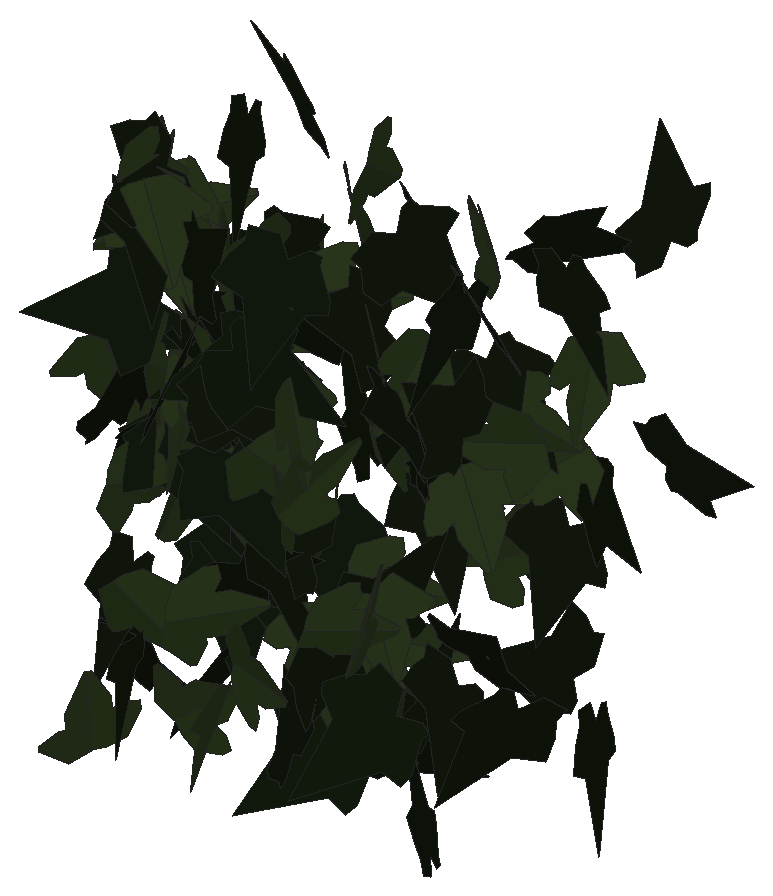
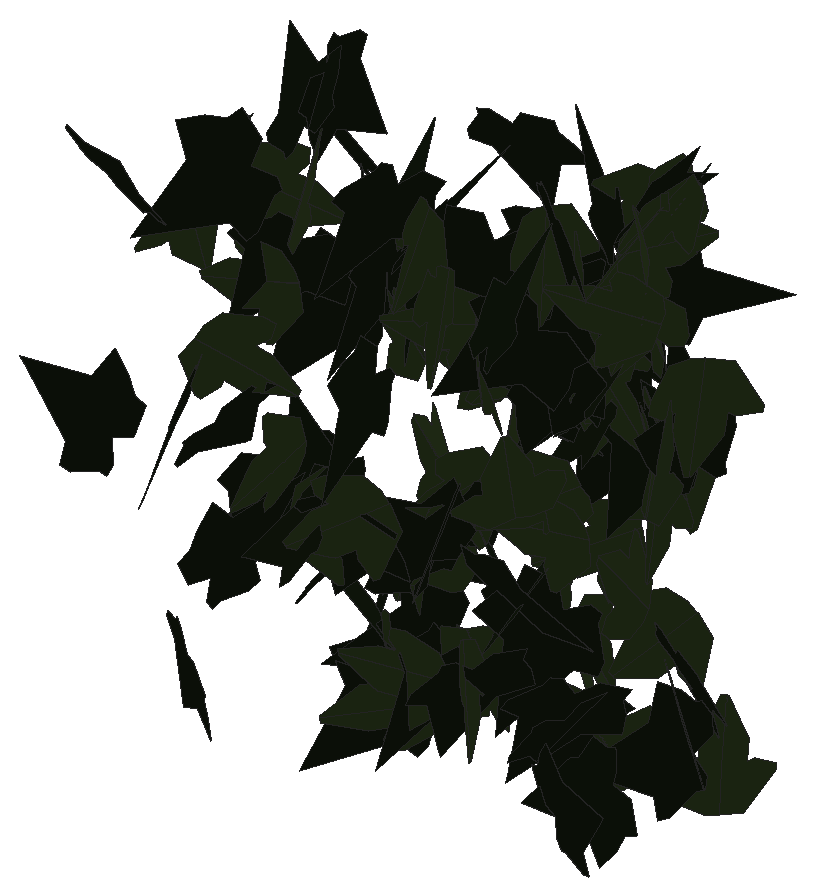
# SketchUp Ruby script. Lengths in inches.
U = 1.inch
M = Sketchup.active_model
def pt(a) = Geom::Point3d.new(a.map { |v| v * U })
def face(e, loops, mat)
  f = e.add_face(loops[0].map { |a| pt(a) })
  loops[1..].each { |l| e.add_face(l.map { |a| pt(a) }).erase! }
  f.material = f.back_material = mat if mat
  f
end
# faces: each face lists its corners as indices into pts; further lists are holes
def faces(e, pts, list, mat = nil) = list.each { |f| face(e, (f[0].is_a?(Array) ? f : [f]).map { |l| l.map { |i| pts[i] } }, mat) }
# xy, xz, yz: faces in a plane at the given z, y or x. An outline is a flat list of corners, or four numbers for a rectangle; further outlines are holes
def ring(l) = l.size == 4 ? [[l[0], l[1]], [l[2], l[1]], [l[2], l[3]], [l[0], l[3]]] : l.each_slice(2).to_a
def flat(e, list, mat, &to3) = list.each { |f| face(e, (f[0].is_a?(Array) ? f : [f]).map { |l| ring(l).map { |u, v| to3.(u, v) } }, mat) }
def xy(e, z, list, mat = nil) = flat(e, list, mat) { |x, y| [x, y, z] }
def xz(e, y, list, mat = nil) = flat(e, list, mat) { |x, z| [x, y, z] }
def yz(e, x, list, mat = nil) = flat(e, list, mat) { |y, z| [x, y, z] }
def lines(e, pts, list) = list.each { |a, b| e.add_line(pt(pts[a]), pt(pts[b])) }
# prism: a flat outline (further loops are holes) pulled along v
def prism(e, loops, v, mat = nil)
  f = face(e, loops, mat); d = Geom::Vector3d.new(v.map { |x| x * U })
  f.pushpull(f.normal.samedirection?(d) ? d.length : -d.length)
end
def box(e, o, s, mat = nil) = prism(e, [[o, [o[0] + s[0], o[1], o[2]], [o[0] + s[0], o[1] + s[1], o[2]], [o[0], o[1] + s[1], o[2]]]], [0, 0, s[2]], mat)
def at(x, y, z, deg = 0) = Geom::Transformation.translation(pt([x, y, z])) * Geom::Transformation.rotation(ORIGIN, Z_AXIS, deg.degrees)
def axes(o, x, y, z) = Geom::Transformation.new([*x, 0, *y, 0, *z, 0, *pt(o).to_a, 1])
def part(name) = M.definitions.add(name)
# library, detail: a bought-in or finely detailed component or shape, given as its bounding box
def library(name, o, s) = part(name).tap { |d| box(d.entities, o, s) }
def detail(e, o, s) = box(e.add_group.entities, o, s)
def put(e, d, t, mat = nil) = e.add_instance(d, t).tap { |i| i.material = mat if mat }
def group(e, t, mat = nil) = e.add_group.tap { |g| g.transformation = t; g.material = mat if mat }.entities
root = M.entities
M.materials.add("efeu1").color = [18, 25, 13]
M.materials.add("efeu2").color = [43, 57, 29]
c1 = part("ivyleaf_10")
p = [[0,0.5,-0.03],[-0.0625,2.02,-0.43],[-0.19,2.01,-0.46],[-0.54,1.05,-0.29],[-0.52,0.625,-0.18],[-0.83,0.76,-0.28],
  [-1.16,0.64,-0.33],[-1.15,0.33,-0.24],[-0.77,-0.39,0.02],[-0.3,-0.51,0.16],[0.04,-0.48,0.23],[-0.02,2.01,-0.4375],
  [-0.06,2.01,-0.43],[0.04,-0.49,0.23],[0.67,-0.49,0.14],[1.38,0.36,-0.2],[1.375,0.51,-0.24],[0.81,0.65,-0.19],
  [0.62,0.59,-0.15],[0.6,1.09,-0.28],[0.5,1.23,-0.31]]
faces(c1.entities,p,[[0,1,2,3,4,5,6,7,8,9,10],[11,12,0,13,14,15,16,17,18,19,20]],"efeu2")
c2 = part("ivyleaf_9")
p = [[1.54,2.16,1.25],[1.36,2.04,1.19],[-0.21,0.99,0.68],[-0.71,1.11,0.82],[-0.85,0.86,0.67],[-0.8,0.17,0.21],
  [-0.9,-0.01,0.1],[-0.67,-0.16,-0.02],[-0.08,-0.08,-0.05],[-0.03,-0.6,-0.4],[0.65,-0.88,-0.66],[0.83,-0.6,-0.49],
  [1.29,-0.42,-0.43],[1.8125,-0.07,-0.26],[1.21,0.44,0.15]]
faces(c2.entities,p,[[0,1,2,3,4,5,6,7,8,9,10,11,12,13,14]],"efeu1")
put(root,c1,axes([36.95,222.88,207.86],[0.184,-0.4165,0.20658],[0.08542,-0.1881,-0.45533],[0.457,0.20285,0.00193]))
put(root,c1,axes([37.33,222.8,208.45],[-0.08205,-0.00713,0.49317],[0.48765,-0.07608,0.08003],[0.0739,0.49413,0.01944]))
put(root,c1,axes([35.91,223.01,211.86],[0.0964,-0.15526,-0.46541],[0.26146,-0.38509,0.18262],[-0.41515,-0.27858,0.00694]))
put(root,c2,axes([35.79,223.12,212.53],[-0.1156,-0.22797,-0.42973],[-0.15203,-0.40263,0.2545],[-0.46208,0.18951,0.02377]))
put(root,c2,axes([37.82,223,213.76],[-0.40431,-0.22695,-0.18715],[0.15558,0.105,-0.46343],[0.24966,-0.43298,-0.01429]))
put(root,c2,axes([40.6,222.65,212.69],[-0.1822,0.25489,0.38966],[-0.26651,0.28602,-0.31171],[-0.38181,-0.32128,0.03164]))
put(root,c1,axes([35.04,223.03,206.71],[-0.22414,-0.4326,-0.11232],[-0.05273,-0.09918,0.48722],[-0.44382,0.23026,-0.00117]))
put(root,c2,axes([36.09,222.89,211.35],[0.01676,0.40736,0.28944],[-0.0313,-0.28818,0.4074],[0.49874,-0.03178,0.01584]))
put(root,c2,axes([39.17,223.2,208.32],[-0.41282,-0.23842,0.1508],[-0.13158,-0.07371,-0.47671],[0.24954,-0.43327,-0.00189]))
put(root,c1,axes([36.69,222.61,209.02],[-0.04745,-0.04622,-0.49559],[0.31785,0.3803,-0.0659],[0.38304,-0.32131,-0.00671]))
put(root,c2,axes([38.24,222.6,207.86],[-0.0403,0.20748,0.45313],[-0.14558,0.42988,-0.20978],[-0.47664,-0.14884,0.02576]))
put(root,c2,axes([35.6,223.27,213.49],[0.08759,-0.46166,0.17087],[0.04316,-0.16568,-0.46977],[0.49037,0.09704,0.01083]))
put(root,c2,axes([37.08,222.98,211.01],[-0.09002,-0.33118,-0.36362],[0.11909,0.34398,-0.34277],[0.47719,-0.14832,0.01695]))
put(root,c2,axes([37.25,222.84,212.48],[0.05635,-0.09212,-0.4882],[0.24441,0.4329,-0.05347],[0.43254,-0.23261,0.09382]))
put(root,c2,axes([39.25,223.34,212.125],[0.33509,-0.32732,-0.17486],[0.1251,-0.12217,0.46843],[-0.34938,-0.35768,0.00001]))
put(root,c2,axes([37.17,222.87,212.18],[-0.05211,-0.22465,-0.44364],[0.10106,0.43197,-0.23062],[0.4869,-0.1137,0.00039]))
put(root,c2,axes([36.38,223.16,213],[-0.08973,0.15688,0.46619],[0.18481,-0.42841,0.17974],[0.45584,0.20457,0.0189]))
put(root,c1,axes([38.91,222.92,209.18],[0.2467,-0.382,0.20788],[-0.1113,0.17559,0.45473],[-0.42042,-0.27064,0.0016]))
put(root,c1,axes([37.58,222.9,211.25],[-0.31894,-0.1942,-0.33251],[0.2846,0.17196,-0.37341],[0.25938,-0.42746,0.00085]))
put(root,c1,axes([37.92,223.04,212.02],[-0.0504,0.49661,-0.02902],[0.00135,-0.02903,-0.49915],[-0.49745,-0.05039,0.00158]))
put(root,c1,axes([36.1875,223.05,211.04],[0.29946,-0.33797,-0.21471],[-0.12996,0.17155,-0.45131],[0.37872,0.32611,0.0149]))
put(root,c2,axes([37.2,222.93,211.44],[-0.25186,-0.14349,0.4074],[0.35402,0.20161,0.28987],[-0.24746,0.43447,0.00005]))
put(root,c1,axes([35.625,222.79,210.31],[-0.06929,-0.13333,-0.47689],[0.20076,0.43262,-0.15012],[0.45265,-0.21229,-0.00642]))
put(root,c1,axes([35.76,223.1,213.79],[0.37441,0.29188,0.15691],[0.12117,0.09978,-0.47472],[-0.30844,0.39351,0.00398]))
put(root,c1,axes([35.56,223.18,210.4375],[0.42739,-0.23548,-0.10903],[0.09637,-0.05104,0.48796],[-0.24094,-0.43811,0.00176]))
put(root,c1,axes([37.61,223.28,210.34],[-0.34031,0.3091,0.19658],[0.14496,-0.13279,0.45973],[0.33641,0.3699,0.00077]))
put(root,c2,axes([38.32,222.97,209],[0.15304,-0.20112,-0.43143],[-0.22958,0.3658,-0.25196],[0.41698,0.27521,0.01963]))
put(root,c2,axes([35.15,223.27,210.77],[0.19529,0.36131,0.28516],[-0.14136,-0.24772,0.41067],[0.43804,-0.24102,0.0054]))
put(root,c2,axes([39.96,223.47,213.85],[-0.12046,0.14245,-0.4639],[0.29865,-0.35497,-0.18655],[-0.38249,-0.32203,0.00044]))
put(root,c2,axes([40.78,223.41,208.86],[-0.0295,0.22699,-0.44453],[0.01659,-0.44461,-0.22813],[-0.49885,-0.02821,0.0187]))
put(root,c1,axes([35.12,223.2,211.6875],[-0.29721,-0.39385,-0.08096],[0.05568,0.05939,-0.49333],[0.39821,-0.30225,0.00855]))
put(root,c1,axes([35.47,223.18,208.61],[-0.37688,-0.00682,-0.32851],[0.32815,0.0177,-0.37683],[0.01677,-0.49964,-0.00887]))
put(root,c1,axes([38.03,222.95,210.8],[0.01219,-0.26064,0.42652],[-0.01608,0.42622,0.26092],[-0.49959,-0.02008,0.002]))
put(root,c2,axes([37.12,223.63,212.06],[-0.03477,-0.16862,-0.46942],[-0.09457,-0.4598,0.17217],[-0.48974,0.10076,0.00008]))
put(root,c2,axes([35.5,223.72,213.875],[-0.12019,-0.33489,0.35129],[-0.12055,-0.32996,-0.3558],[0.47013,-0.17022,-0.00143]))
put(root,c1,axes([38.33,223,209.26],[-0.10549,-0.13096,-0.47087],[0.27074,0.3854,-0.16784],[0.40691,-0.29038,-0.0104]))
put(root,c2,axes([35.17,223.53,207.88],[-0.2336,-0.01165,-0.44192],[0.43392,-0.10162,-0.22669],[-0.08454,-0.48943,0.05758]))
put(root,c2,axes([36.01,223.29,210.87],[-0.09702,-0.31256,-0.37801],[0.11921,0.35876,-0.32723],[0.47579,-0.15362,0.00491]))
put(root,c1,axes([35.55,223.71,213.34],[-0.01621,-0.02466,0.49913],[-0.01783,-0.49904,-0.02524],[0.49942,-0.01861,0.0153]))
put(root,c2,axes([38.12,223.65,207.41],[-0.39095,-0.22807,0.21247],[-0.17215,-0.12614,-0.45216],[0.25986,-0.4267,0.02011]))
put(root,c2,axes([39.67,223.25,206.81],[0.00632,-0.29978,0.40011],[-0.02204,0.39959,0.29974],[-0.49947,-0.02143,-0.00816]))
put(root,c2,axes([39.15,223.66,211.52],[-0.06816,0.10495,0.48409],[0.12821,-0.46826,0.11957],[0.47845,0.14042,0.03692]))
put(root,c1,axes([40.8,223.51,212.28],[0.11605,0.0432,-0.48442],[-0.48634,0.01101,-0.11553],[0.00069,0.49801,0.04457]))
put(root,c1,axes([35.57,223.3125,210.3],[0.04062,-0.39502,-0.30382],[-0.03298,0.30203,-0.3971],[0.49725,0.0523,-0.00152]))
put(root,c2,axes([35.05,223.6875,208.6],[-0.40034,-0.00903,-0.29941],[0.29939,-0.02827,-0.39946],[-0.00972,-0.49912,0.02805]))
put(root,c2,axes([35.73,223.18,210.98],[0.14673,0.45014,0.16076],[0.04454,0.15456,-0.47342],[-0.47591,0.15325,0.00526]))
put(root,c1,axes([35.4,223.21,213.94],[-0.04742,-0.18683,-0.46135],[0.13488,0.44128,-0.19257],[0.47912,-0.14271,0.00855]))
put(root,c2,axes([40,223.86,213.45],[-0.02815,-0.21384,0.45109],[0.21252,-0.41395,-0.18297],[0.45171,0.18143,0.11419]))
put(root,c1,axes([36.15,223.21,211.19],[0.09944,0.16868,-0.46007],[0.0979,0.45314,0.1873],[0.48013,-0.12733,0.05709]))
put(root,c1,axes([35.89,223.62,207.01],[-0.32824,-0.09048,0.36616],[0.35585,0.08661,0.34039],[-0.12502,0.48406,0.00754]))
put(root,c1,axes([38.4,223.3,208.02],[0.05816,0.25341,-0.42708],[0.04944,0.42491,0.25886],[0.49414,-0.07234,0.02437]))
put(root,c1,axes([36.18,223.66,211.63],[-0.29461,0.02072,0.40346],[-0.40301,-0.04971,-0.29173],[0.02802,-0.49709,0.04599]))
put(root,c2,axes([38.32,224.06,212.67],[0.12636,-0.44327,-0.19377],[0.05701,-0.18523,0.46091],[-0.4804,-0.13858,0.00373]))
put(root,c2,axes([36.02,223.68,211.34],[0.40596,-0.28212,-0.07488],[-0.06115,0.04322,-0.49436],[0.28541,0.41054,0.00058]))
put(root,c2,axes([39.43,224.05,208.41],[-0.00297,-0.45159,0.21461],[0.01468,-0.2146,-0.45137],[0.49978,0.00362,0.01453]))
put(root,c2,axes([36,224.07,211.51],[0.31207,-0.36889,-0.12856],[0.08244,-0.09865,0.48319],[-0.38186,-0.32278,-0.00075]))
put(root,c2,axes([34.9,223.71,207.48],[0.41265,-0.12606,0.25264],[0.24056,-0.07724,-0.43147],[0.14782,0.47764,-0.0031]))
put(root,c1,axes([39.88,223.66,211.32],[0.30403,0.37276,0.13644],[0.08607,0.10587,-0.48102],[-0.3875,0.31598,0.00021]))
put(root,c1,axes([39.01,223.95,212.58],[0.14434,0.34728,-0.32949],[-0.14204,-0.29757,-0.37587],[-0.45715,0.20211,0.01275]))
put(root,c2,axes([36.62,223.95,211.625],[-0.13008,0.2527,-0.41136],[0.18734,-0.36623,-0.28422],[-0.44495,-0.22807,0.0006]))
put(root,c1,axes([35.18,223.91,210.62],[-0.39338,0.27809,0.13386],[0.10223,-0.08721,0.48161],[0.2912,0.40628,0.01176]))
put(root,c1,axes([38.4,224.05,211.39],[0.15473,-0.10861,-0.46289],[0.36902,-0.27951,0.18893],[-0.2998,-0.4001,-0.00634]))
put(root,c2,axes([39.6,224.06,208.9],[0.48632,-0.0342,-0.11102],[0.11068,-0.00886,0.48752],[-0.03531,-0.49875,-0.00105]))
put(root,c1,axes([36.7,223.85,213.27],[-0.09785,-0.47618,-0.11696],[0.03257,0.11269,-0.48605],[0.48925,-0.10274,0.00896]))
put(root,c1,axes([35.6875,224.13,213.08],[-0.19854,0.35363,0.29246],[-0.00289,-0.31961,0.3845],[0.45888,0.15099,0.12896]))
put(root,c2,axes([38.49,223.77,212.62],[0.23413,-0.028,-0.4409],[-0.42861,0.10661,-0.23437],[0.10714,0.4877,0.02592]))
put(root,c1,axes([35.93,224.17,212.89],[0.22182,-0.13595,0.42698],[0.38721,-0.18164,-0.25899],[0.22554,0.44556,0.02469]))
put(root,c2,axes([37.55,223.73,212.74],[0.2309,0.44065,-0.0501],[-0.02305,-0.04449,-0.49748],[-0.44289,0.23205,-0.00023]))
put(root,c1,axes([38.34,223.92,209.17],[0.19691,0.44845,0.10059],[0.0415,0.09164,-0.48978],[-0.45772,0.20123,-0.00113]))
put(root,c2,axes([39.53,223.71,211.59],[0.33493,0.35751,0.10005],[0.06891,0.07254,-0.48989],[-0.36479,0.34194,-0.00068]))
put(root,c1,axes([35.29,223.97,212.875],[0.38847,0.24896,0.19264],[0.15807,0.11033,-0.46135],[-0.27222,0.41934,0.00701]))
put(root,c2,axes([38.03,223.77,207.93],[0.09498,0.07526,-0.48509],[0.19151,0.44926,0.1072],[0.452,-0.20616,0.05652]))
put(root,c2,axes([38.82,223.8,212.18],[0.1059,-0.16651,-0.45941],[-0.24499,0.38864,-0.19733],[0.42281,0.2669,0.00073]))
put(root,c2,axes([36.0625,224.03,211.98],[0.17431,0.07333,-0.46286],[0.41051,0.21431,0.18855],[0.22605,-0.44575,0.01451]))
put(root,c1,axes([35.46,223.92,209.27],[0.15371,-0.37332,0.29496],[-0.11442,0.27187,0.40373],[-0.46182,-0.19161,-0.00185]))
put(root,c1,axes([36.24,224.125,209.84],[-0.06084,-0.04738,-0.49402],[0.49226,-0.06901,-0.054],[-0.06307,-0.49294,0.05504]))
put(root,c2,axes([38.95,223.86,207.75],[-0.34632,0.36035,-0.01465],[-0.01552,0.0054,0.49973],[0.36031,0.34658,0.00744]))
put(root,c1,axes([37.23,224.3,207.875],[0.37149,-0.13056,0.30814],[0.28664,-0.11346,-0.39365],[0.17271,0.46913,-0.00945]))
put(root,c2,axes([36.61,224.32,209.08],[0.22596,-0.44308,0.05121],[0.02377,-0.04537,-0.49737],[0.4454,0.2272,0.00056]))
put(root,c2,axes([38.24,223.95,208.8125],[-0.07249,-0.11008,0.48232],[0.41213,0.25622,0.12042],[-0.27367,0.41501,0.05359]))
put(root,c1,axes([35.25,224.02,213.41],[0.14908,-0.1154,0.4631],[-0.3704,0.27797,0.1885],[-0.30096,-0.39927,-0.00261]))
put(root,c1,axes([37.24,224.36,208.28],[0.47353,0.12268,-0.10355],[-0.10328,-0.01412,-0.48901],[-0.12291,0.48451,0.01197]))
put(root,c1,axes([36.32,224.11,210.34],[0.16944,0.14248,0.44832],[0.3181,0.31634,-0.22076],[-0.34655,0.36004,0.01656]))
put(root,c2,axes([36.31,224.13,208.875],[0.33681,0.36945,0.00787],[0.00351,0.00745,-0.49993],[-0.36952,0.33682,0.00242]))
put(root,c2,axes([38.39,224.11,207.28],[0.37424,0.27529,0.18483],[0.14704,0.11202,-0.46458],[-0.29719,0.40208,0.00289]))
put(root,c1,axes([38.58,224.1,207.46],[0.02838,-0.05027,0.49666],[-0.28622,0.40593,0.05744],[-0.40899,-0.28756,-0.00574]))
put(root,c1,axes([35.15,224.27,212.93],[0.13353,0.03475,-0.48059],[0.45262,0.16199,0.13747],[0.16526,-0.47175,0.0118]))
put(root,c2,axes([35.67,224.09,206.99],[-0.13357,0.36783,-0.31122],[-0.14318,0.27807,0.3901],[0.46006,0.19333,0.03105]))
put(root,c2,axes([36.97,224.44,209.1],[-0.30615,0.17285,0.35552],[-0.30769,0.17811,-0.35157],[-0.24818,-0.43405,-0.00269]))
put(root,c2,axes([39.53,224.51,212.42],[-0.12399,-0.20414,-0.43926],[0.21671,0.38213,-0.23876],[0.4332,-0.2496,-0.00628]))
put(root,c1,axes([39.74,224.64,211.92],[-0.14108,0.00102,-0.47968],[0.47068,-0.09612,-0.13864],[-0.0925,-0.49067,0.02616]))
put(root,c2,axes([35.82,224.8,214.11],[-0.2904,0.01868,-0.4066],[0.40441,-0.04329,-0.29082],[-0.04607,-0.49777,0.01003]))
put(root,c2,axes([40.24,225.07,208.41],[0.01062,-0.00918,0.4998],[-0.33359,-0.37245,0.00025],[0.3723,-0.33346,-0.01404]))
put(root,c2,axes([40.19,225.08,210.26],[-0.08322,-0.47658,0.12627],[-0.02538,-0.12374,-0.48378],[0.49237,-0.08693,-0.00359]))
put(root,c2,axes([38.2,224.56,213.5625],[0.0422,-0.21512,-0.44938],[-0.0911,0.44006,-0.21921],[0.48982,0.10038,-0.00205]))
put(root,c2,axes([35.55,224.97,208.2],[-0.05388,-0.48769,-0.09621],[0.01146,0.09553,-0.49066],[0.49696,-0.05508,0.00088]))
put(root,c1,axes([36.97,224.71,212.39],[0.01011,-0.06243,-0.49598],[0.47785,0.14691,-0.00875],[0.14683,-0.47383,0.06263]))
put(root,c1,axes([40.19,225.09,211.18],[0.26509,0.12645,-0.40465],[-0.37533,-0.15191,-0.29335],[-0.19712,0.45928,0.01439]))
put(root,c1,axes([40.61,225.02,212.7],[0.18173,0.44165,-0.14805],[-0.05634,-0.13691,-0.47758],[-0.46238,0.19027,0]))
put(root,c2,axes([36.08,224.84,212.68],[-0.04998,-0.05865,-0.49403],[0.27754,0.40878,-0.07661],[0.41288,-0.28188,-0.0083]))
put(root,c1,axes([39.61,224.62,209.87],[-0.02787,0.08716,0.49156],[-0.12683,0.47493,-0.0914],[-0.48284,-0.12978,-0.00437]))
put(root,c2,axes([35.46,224.97,208.53],[-0.0221,-0.33617,-0.36946],[0.08949,0.36117,-0.33399],[0.49143,-0.08089,0.04421]))
put(root,c2,axes([40.12,225.18,213.49],[0.22438,-0.44613,0.02491],[0.01339,-0.02115,-0.49937],[0.44662,0.22477,0.00246]))
put(root,c1,axes([38.95,225.24,213.2],[-0.30811,0.3799,0.10364],[0.05942,-0.08523,0.48909],[0.38928,0.3137,0.00738]))
put(root,c2,axes([37.375,224.85,208.25],[-0.00831,0.01589,-0.49968],[-0.30162,0.39839,0.01768],[0.3987,0.30172,0.00296]))
put(root,c1,axes([36.26,225.49,212.4],[0.30408,-0.22211,0.32894],[0.27846,-0.1759,-0.37619],[0.28284,0.41197,0.01672]))
put(root,c1,axes([38.76,225.26,209.63],[-0.16412,0.09715,-0.4622],[-0.44788,0.12328,0.18495],[0.14989,0.47473,0.04656]))
put(root,c2,axes([40.25,225.51,207.57],[-0.21253,-0.00744,-0.45252],[0.45178,-0.03324,-0.21164],[-0.02693,-0.49884,0.02085]))
put(root,c2,axes([38.1,225.44,209.96],[-0.29313,-0.18451,-0.36059],[0.3141,0.1775,-0.34617],[0.25575,-0.42948,0.01185]))
put(root,c1,axes([37.43,225.16,207.84],[0.05132,0.0408,0.49568],[0.31263,0.38491,-0.06405],[-0.38682,0.31651,0.014]))
put(root,c1,axes([37.1,225.42,208.39],[0.00546,-0.02008,-0.49957],[0.49987,-0.00974,0.00585],[-0.00997,-0.4995,0.01997]))
put(root,c2,axes([40.38,225.3,210.77],[0.28165,-0.20238,-0.36016],[-0.29176,0.21117,-0.34682],[0.29249,0.40552,0.00086]))
put(root,c2,axes([35.42,225.28,207.24],[-0.03077,0.03968,0.49747],[-0.25891,0.42482,-0.0499],[-0.42664,-0.26067,-0.00559]))
put(root,c2,axes([36.32,225.6,208.8],[-0.05137,-0.43447,-0.24206],[0.02826,0.24041,-0.4375],[0.49655,-0.05863,-0.00014]))
put(root,c2,axes([38.41,225.64,209.91],[0.36099,-0.33138,0.09935],[0.07683,-0.06322,-0.49],[0.33732,0.36904,0.00528]))
put(root,c1,axes([37.84,225.49,210.16],[-0.27766,-0.03345,-0.41447],[0.40979,0.06251,-0.27958],[0.07052,-0.49495,-0.0073]))
put(root,c1,axes([37.16,225.34,213.79],[0.01203,-0.30079,-0.39922],[-0.00136,0.39932,-0.30091],[0.49985,0.00833,0.00878]))
put(root,c1,axes([36.87,225.45,213.17],[-0.38723,0.24456,0.2006],[-0.16455,0.11506,-0.45791],[-0.27013,-0.42066,-0.00863]))
put(root,c2,axes([39.61,225.32,213.66],[0.32426,0.26536,0.27283],[0.19907,0.18723,-0.41871],[-0.32438,0.38017,0.01577]))
put(root,c2,axes([36.9,225.61,209.93],[-0.01177,-0.34952,0.35735],[0.01065,0.35719,0.34971],[-0.49975,0.01584,-0.00096]))
put(root,c1,axes([36.38,225.59,208.875],[0.15031,-0.42296,-0.22026],[-0.05772,0.21311,-0.44861],[0.47337,0.16029,0.01524]))
put(root,c1,axes([35.72,225.62,211.07],[0.29721,0.3856,-0.11392],[0.05741,0.09951,0.48662],[0.39796,-0.30233,0.01488]))
put(root,c2,axes([35.49,226.33,213.45],[0.21679,-0.41664,0.1715],[-0.06579,0.15901,0.46945],[-0.44573,-0.22611,0.01412]))
put(root,c2,axes([40.55,226.48,210.61],[0.13897,-0.11442,0.46647],[0.37808,-0.27343,-0.1797],[0.29622,0.40267,0.01052]))
put(root,c2,axes([40.67,226.33,213.67],[-0.46436,0.12353,-0.13823],[-0.13356,0.03562,0.48051],[0.12856,0.48319,-0.00008]))
put(root,c2,axes([36.93,226.53,212.56],[0.42612,-0.04453,-0.25776],[-0.25506,0.03859,-0.42832],[0.05804,0.49652,0.01017]))
